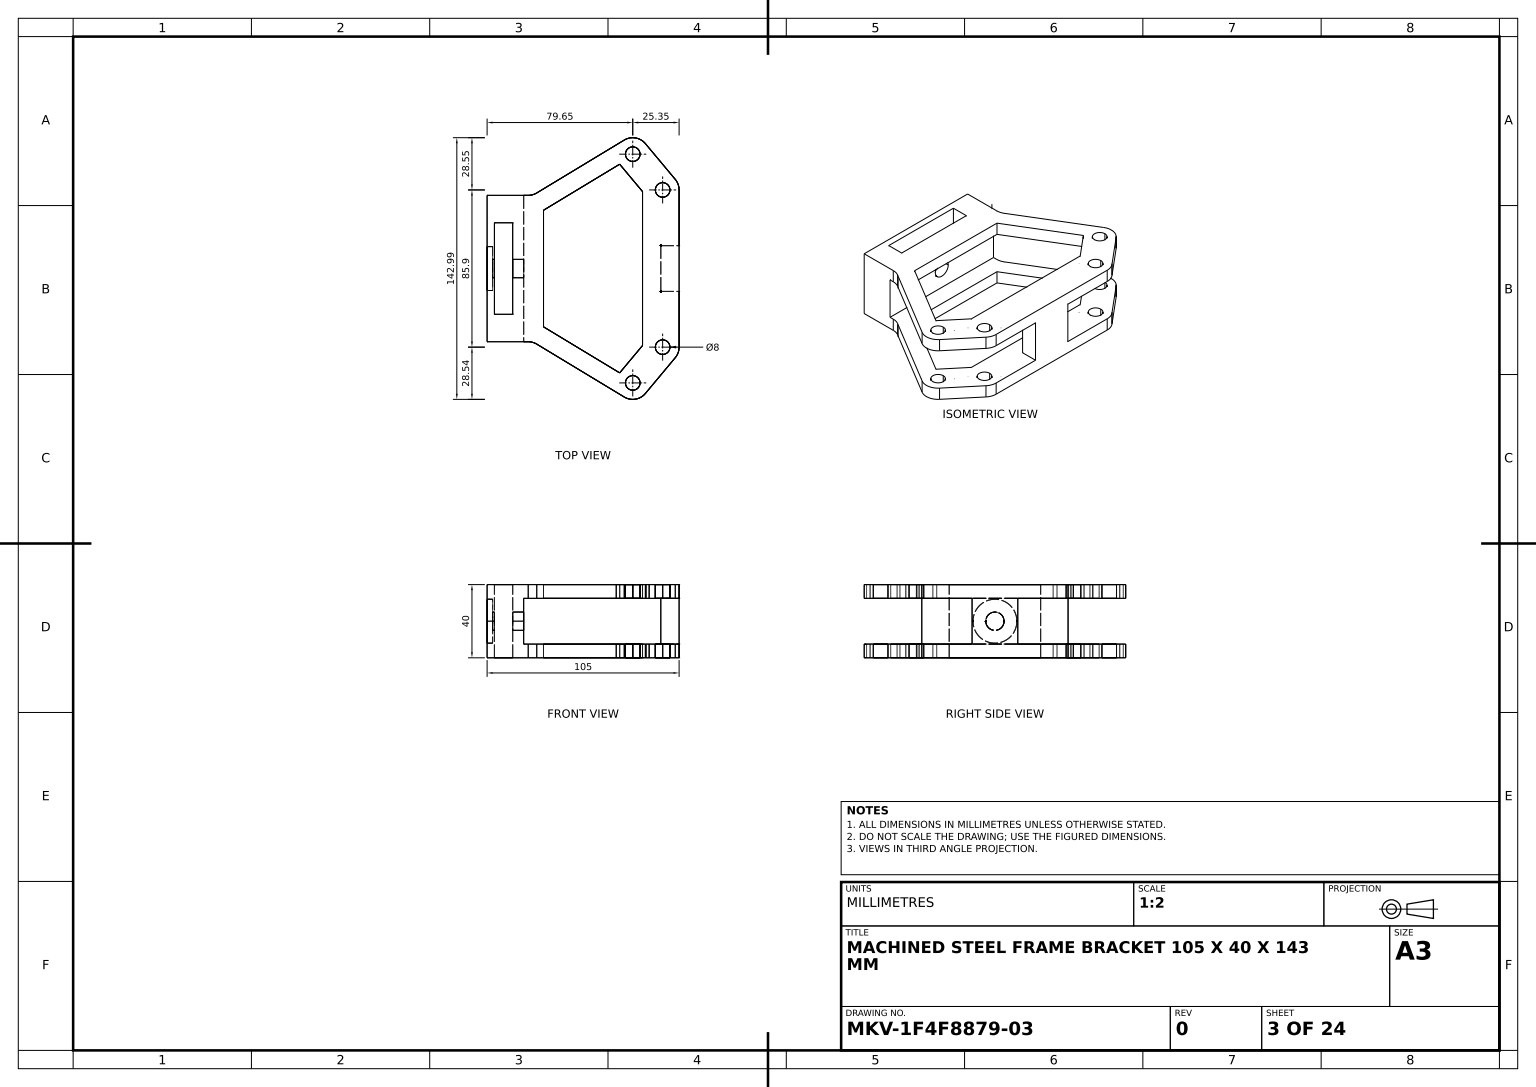
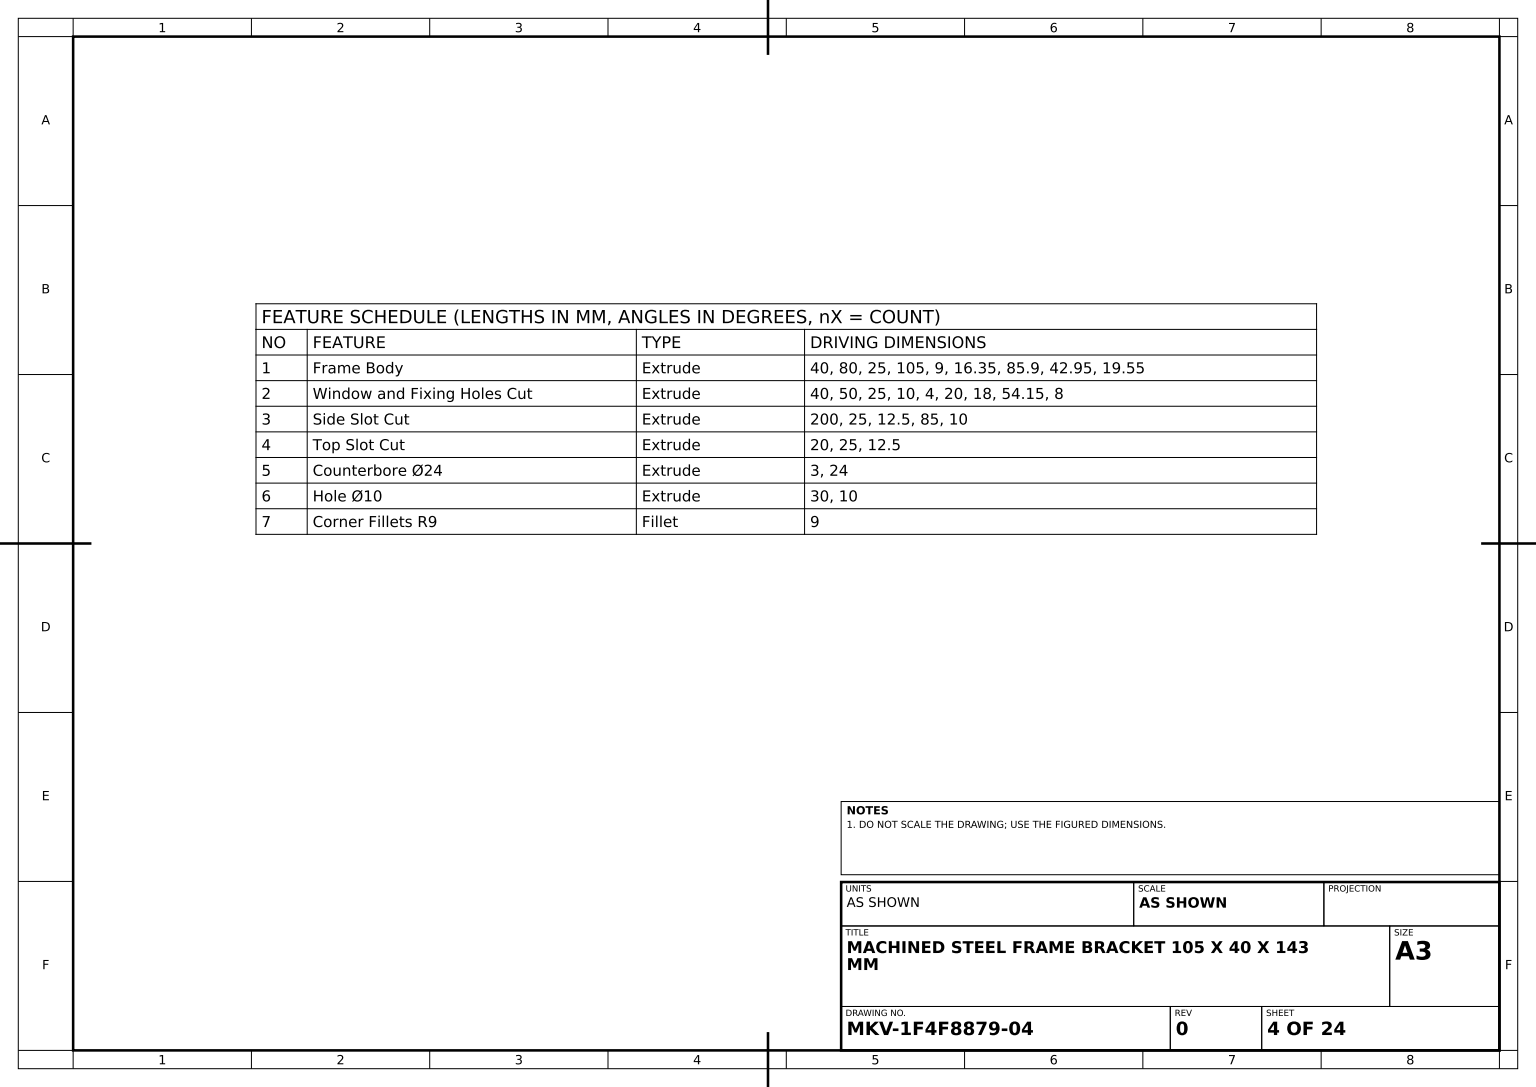
solid
v1 (27.146251,-12.5,-41.296579)
v2 (22.492509,-12.5,-40)
e1 v1 v2 CIRCLE(AX(P(22.492509,-12.5,-49),D(0,-1,0),D(0,0,-1)),9)
v3 (27.146251,-20,-41.296579)
e2 v3 v1 LINE
v4 (22.492509,-20,-40)
e3 v4 v3 CIRCLE(AX(P(22.492509,-20,-49),D(0,1,0),D(0,0,-1)),9)
e4 v2 v4 LINE
face CYL(AX(P(22.492509,20,-49),D(0,1,0),D(0,0,1)),9) rev [-e1 -e2 -e3 -e4]
v5 (95,-12.5,-12.5)
v6 (95,-12.5,12.5)
e5 v5 v6 LINE
v7 (95,12.5,12.5)
e6 v6 v7 LINE
v8 (95,12.5,-12.5)
e7 v8 v7 LINE
e8 v8 v5 LINE
face PLANE(AX(P(95,12.5,-100),D(1,0,0),D(0,1,0))) rev [e5 e6 -e7 e8]
v9 (79.65,-12.5,58.5)
v10 (79.65,-12.5,66.5)
e9 v9 v10 CIRCLE(AX(P(79.65,-12.5,62.5),D(0,1,0),D(0,0,-1)),4)
v11 (79.65,-20,66.5)
e10 v11 v10 LINE
v12 (79.65,-20,58.5)
e11 v12 v11 CIRCLE(AX(P(79.65,-20,62.5),D(0,1,0),D(0,0,1)),4)
e12 v12 v9 LINE
face CYL(AX(P(79.65,-20,62.5),D(0,1,0),D(0,0,1)),4) rev [e9 -e10 -e11 e12]
v13 (86.55385,-12.5,-68.273808)
v14 (86.55385,-20,-68.273808)
e13 v13 v14 LINE
v15 (79.65,-20,-71.5)
e14 v14 v15 CIRCLE(AX(P(79.65,-20,-62.5),D(0,1,0),D(0,0,1)),9)
v16 (79.65,-12.5,-71.5)
e15 v16 v15 LINE
e16 v16 v13 CIRCLE(AX(P(79.65,-12.5,-62.5),D(0,-1,0),D(0,0,-1)),9)
face CYL(AX(P(79.65,20,-62.5),D(0,-1,0),D(0,0,-1)),9) [e13 e14 -e15 e16]
v17 (0,0,-12)
v18 (0,0,12)
e17 v17 v18 CIRCLE(AX(P(0,0,0),D(-1,0,0),D(0,0,1)),12)
v19 (3,0,12)
e18 v19 v18 LINE
v20 (3,0,-12)
e19 v20 v19 CIRCLE(AX(P(3,0,0),D(-1,0,0),D(0,0,1)),12)
e20 v20 v17 LINE
face CYL(AX(P(3,0,0),D(-1,0,0),D(0,0,1)),12) rev [e17 -e18 -e19 e20]
v21 (86.55385,-12.5,68.273808)
v22 (74.996259,-12.5,70.203421)
e21 v21 v22 CIRCLE(AX(P(79.65,-12.5,62.5),D(0,-1,0),D(0,0,-1)),9)
v23 (74.996259,-20,70.203421)
e22 v22 v23 LINE
v24 (86.55385,-20,68.273808)
e23 v23 v24 CIRCLE(AX(P(79.65,-20,62.5),D(0,1,0),D(0,0,-1)),9)
e24 v21 v24 LINE
face CYL(AX(P(79.65,20,62.5),D(0,-1,0),D(0,0,-1)),9) [e21 e22 e23 -e24]
v25 (96,20,-46.95)
v26 (96,20,-38.95)
e25 v25 v26 CIRCLE(AX(P(96,20,-42.95),D(0,1,0),D(0,0,1)),4)
v27 (96,12.5,-38.95)
e26 v27 v26 LINE
v28 (96,12.5,-46.95)
e27 v27 v28 CIRCLE(AX(P(96,12.5,-42.95),D(0,-1,0),D(0,0,1)),4)
e28 v28 v25 LINE
face CYL(AX(P(96,-20,-42.95),D(0,1,0),D(0,0,1)),4) rev [e25 -e26 e27 e28]
v29 (105,-12.5,12.5)
e29 v6 v29 LINE
v30 (105,12.5,12.5)
e30 v29 v30 LINE
e31 v7 v30 LINE
face PLANE(AX(P(85,12.5,12.5),D(0,0,-1),D(-1,0,0))) rev [e29 e30 -e31 -e6]
e32 v11 v12 CIRCLE(AX(P(79.65,-20,62.5),D(0,1,0),D(0,0,1)),4)
e33 v10 v9 CIRCLE(AX(P(79.65,-12.5,62.5),D(0,1,0),D(0,0,-1)),4)
face CYL(AX(P(79.65,-20,62.5),D(0,1,0),D(0,0,1)),4) rev [-e12 -e32 e10 e33]
v31 (105,20,-42.95)
v32 (102.90385,20,-48.723808)
e34 v31 v32 CIRCLE(AX(P(96,20,-42.95),D(0,1,0),D(0,0,-1)),9)
v33 (105,12.5,-42.95)
e35 v31 v33 LINE
v34 (102.90385,12.5,-48.723808)
e36 v33 v34 CIRCLE(AX(P(96,12.5,-42.95),D(0,1,0),D(0,0,1)),9)
e37 v32 v34 LINE
face CYL(AX(P(96,20,-42.95),D(0,-1,0),D(0,0,-1)),9) [-e34 e35 e36 -e37]
v35 (74.996259,20,70.203421)
v36 (86.55385,20,68.273808)
e38 v35 v36 CIRCLE(AX(P(79.65,20,62.5),D(0,1,0),D(0,0,-1)),9)
v37 (74.996259,12.5,70.203421)
e39 v35 v37 LINE
v38 (86.55385,12.5,68.273808)
e40 v37 v38 CIRCLE(AX(P(79.65,12.5,62.5),D(0,1,0),D(0,0,1)),9)
e41 v36 v38 LINE
face CYL(AX(P(79.65,20,62.5),D(0,-1,0),D(0,0,-1)),9) [-e38 e39 e40 -e41]
v39 (0,20,-40)
v40 (0,-20,-40)
e42 v39 v40 LINE
v41 (22.492509,20,-40)
e43 v41 v39 LINE
v42 (22.492509,12.5,-40)
e44 v41 v42 LINE
v43 (20,12.5,-40)
e45 v42 v43 LINE
v44 (20,-12.5,-40)
e46 v43 v44 LINE
e47 v44 v2 LINE
e48 v4 v40 LINE
face PLANE(AX(P(0,20,-40),D(0,0,1),D(1,0,0))) rev [-e42 -e43 e44 e45 e46 e47 e4 e48]
v45 (79.65,20,66.5)
v46 (79.65,20,58.5)
e49 v45 v46 CIRCLE(AX(P(79.65,20,62.5),D(0,1,0),D(0,0,1)),4)
v47 (79.65,12.5,58.5)
e50 v47 v46 LINE
v48 (79.65,12.5,66.5)
e51 v47 v48 CIRCLE(AX(P(79.65,12.5,62.5),D(0,-1,0),D(0,0,1)),4)
e52 v48 v45 LINE
face CYL(AX(P(79.65,-20,62.5),D(0,1,0),D(0,0,1)),4) rev [e49 -e50 e51 e52]
v49 (79.65,20,-71.5)
v50 (79.65,12.5,-71.5)
e53 v49 v50 LINE
v51 (74.996259,12.5,-70.203421)
e54 v50 v51 CIRCLE(AX(P(79.65,12.5,-62.5),D(0,1,0),D(0,0,1)),9)
v52 (74.996259,20,-70.203421)
e55 v52 v51 LINE
e56 v49 v52 CIRCLE(AX(P(79.65,20,-62.5),D(0,1,0),D(0,0,1)),9)
face CYL(AX(P(79.65,20,-62.5),D(0,-1,0),D(0,0,-1)),9) [e53 e54 -e55 -e56]
v53 (102.90385,-20,48.723808)
e57 v24 v53 LINE
v54 (102.90385,-12.5,48.723808)
e58 v54 v53 LINE
e59 v54 v21 LINE
face PLANE(AX(P(102.90385,20,48.723808),D(-0.767094424,0,-0.641534211),D(-0.641534211,0,0.767094424))) rev [e57 -e58 e59 e24]
v55 (14,20,-25)
v56 (4,20,-25)
e60 v55 v56 LINE
v57 (4,-20,-25)
e61 v57 v56 LINE
v58 (14,-20,-25)
e62 v58 v57 LINE
e63 v58 v55 LINE
face PLANE(AX(P(4,-20,-25),D(0,0,-1),D(-1,0,0))) rev [e60 -e61 -e62 e63]
v59 (105,12.5,-12.5)
v60 (105,-12.5,-12.5)
e64 v59 v60 LINE
e65 v33 v59 LINE
v61 (105,20,42.95)
e66 v61 v31 LINE
v62 (105,12.5,42.95)
e67 v61 v62 LINE
e68 v30 v62 LINE
v63 (105,-12.5,42.95)
e69 v63 v29 LINE
v64 (105,-20,42.95)
e70 v63 v64 LINE
v65 (105,-20,-42.95)
e71 v64 v65 LINE
v66 (105,-12.5,-42.95)
e72 v66 v65 LINE
e73 v60 v66 LINE
face PLANE(AX(P(105,20,-42.95),D(-1,0,0),D(0,0,1))) rev [-e64 -e65 -e35 -e66 e67 -e68 -e30 -e69 e70 e71 -e72 -e73]
v67 (86.55385,20,-68.273808)
e74 v67 v49 CIRCLE(AX(P(79.65,20,-62.5),D(0,1,0),D(0,0,1)),9)
v68 (86.55385,12.5,-68.273808)
e75 v67 v68 LINE
e76 v68 v50 CIRCLE(AX(P(79.65,12.5,-62.5),D(0,1,0),D(0,0,1)),9)
face CYL(AX(P(79.65,20,-62.5),D(0,-1,0),D(0,0,-1)),9) [-e74 e75 e76 -e53]
v69 (30.85,-20,31.850943)
v70 (30.85,-12.5,31.850943)
e77 v69 v70 LINE
v71 (30.85,-20,-31.850943)
e78 v71 v69 LINE
v72 (30.85,-12.5,-31.850943)
e79 v71 v72 LINE
e80 v72 v70 LINE
face PLANE(AX(P(30.85,-20,-31.850943),D(-1,0,0),D(0,0,1))) rev [-e77 -e78 e79 e80]
v73 (4,0,5)
v74 (4,0,-5)
e81 v73 v74 CIRCLE(AX(P(4,0,0),D(-1,0,0),D(0,0,1)),5)
v75 (3,0,5)
e82 v73 v75 LINE
v76 (3,0,-5)
e83 v75 v76 CIRCLE(AX(P(3,0,0),D(-1,0,0),D(0,0,1)),5)
e84 v74 v76 LINE
face CYL(AX(P(33,0,0),D(-1,0,0),D(0,0,1)),5) rev [-e81 e82 e83 -e84]
v77 (85,-20,42.074035)
v78 (85,-20,-42.074035)
e85 v77 v78 LINE
v79 (85,-12.5,42.074035)
e86 v77 v79 LINE
v80 (85,-12.5,-42.074035)
e87 v79 v80 LINE
e88 v78 v80 LINE
face PLANE(AX(P(85,-20,42.074035),D(1,0,0),D(0,0,-1))) rev [-e85 e86 e87 -e88]
v81 (96,-20,-46.95)
v82 (96,-20,-38.95)
e89 v81 v82 CIRCLE(AX(P(96,-20,-42.95),D(0,1,0),D(0,0,1)),4)
e90 v82 v81 CIRCLE(AX(P(96,-20,-42.95),D(0,1,0),D(0,0,1)),4)
v83 (79.65,-20,-58.5)
v84 (79.65,-20,-66.5)
e91 v83 v84 CIRCLE(AX(P(79.65,-20,-62.5),D(0,1,0),D(0,0,1)),4)
e92 v84 v83 CIRCLE(AX(P(79.65,-20,-62.5),D(0,1,0),D(0,0,1)),4)
v85 (72.50458,-20,-57.015042)
e93 v78 v85 LINE
e94 v85 v71 LINE
v86 (72.50458,-20,57.015042)
e95 v69 v86 LINE
e96 v86 v77 LINE
v87 (4,-20,25)
e97 v57 v87 LINE
v88 (14,-20,25)
e98 v87 v88 LINE
e99 v88 v58 LINE
v89 (96,-20,46.95)
v90 (96,-20,38.95)
e100 v89 v90 CIRCLE(AX(P(96,-20,42.95),D(0,1,0),D(0,0,1)),4)
e101 v90 v89 CIRCLE(AX(P(96,-20,42.95),D(0,1,0),D(0,0,1)),4)
e102 v53 v64 CIRCLE(AX(P(96,-20,42.95),D(0,1,0),D(0,0,-1)),9)
v91 (27.146251,-20,41.296579)
e103 v91 v23 LINE
v92 (22.492509,-20,40)
e104 v91 v92 CIRCLE(AX(P(22.492509,-20,49),D(0,1,0),D(0,0,-1)),9)
v93 (0,-20,40)
e105 v93 v92 LINE
e106 v40 v93 LINE
v94 (74.996259,-20,-70.203421)
e107 v94 v3 LINE
e108 v15 v94 CIRCLE(AX(P(79.65,-20,-62.5),D(0,1,0),D(0,0,1)),9)
v95 (102.90385,-20,-48.723808)
e109 v95 v14 LINE
e110 v65 v95 CIRCLE(AX(P(96,-20,-42.95),D(0,1,0),D(0,0,-1)),9)
face PLANE(AX(P(79.65,-20,62.5),D(0,-1,0),D(0,0,-1))) [e89 e90] [e91 e92] [e11 e32] [e93 e94 e78 e95 e96 e85] [e62 e97 e98 e99] [e100 e101] [-e102 -e57 -e23 -e103 e104 -e105 -e106 -e48 e3 -e107 -e108 -e14 -e109 -e110 -e71]
e111 v74 v73 CIRCLE(AX(P(4,0,0),D(-1,0,0),D(0,0,1)),5)
v96 (4,20,25)
e112 v56 v96 LINE
e113 v87 v96 LINE
face PLANE(AX(P(4,-20,-25),D(-1,0,0),D(0,0,1))) rev [e81 e111] [-e97 e61 e112 -e113]
v97 (74.996259,-12.5,-70.203421)
e114 v97 v94 LINE
e115 v1 v97 LINE
face PLANE(AX(P(25,20,-40),D(0.517082376,0,0.855935638),D(0.855935638,0,-0.517082376))) rev [e114 e107 e2 e115]
v98 (79.65,12.5,-66.5)
v99 (79.65,20,-66.5)
e116 v98 v99 LINE
v100 (79.65,20,-58.5)
e117 v99 v100 CIRCLE(AX(P(79.65,20,-62.5),D(0,1,0),D(0,0,1)),4)
v101 (79.65,12.5,-58.5)
e118 v101 v100 LINE
e119 v101 v98 CIRCLE(AX(P(79.65,12.5,-62.5),D(0,-1,0),D(0,0,1)),4)
face CYL(AX(P(79.65,-20,-62.5),D(0,1,0),D(0,0,1)),4) rev [e116 e117 -e118 e119]
v102 (22.492509,-12.5,40)
e120 v92 v102 LINE
v103 (27.146251,-12.5,41.296579)
e121 v103 v91 LINE
e122 v102 v103 CIRCLE(AX(P(22.492509,-12.5,49),D(0,-1,0),D(0,0,-1)),9)
face CYL(AX(P(22.492509,20,49),D(0,1,0),D(0,0,1)),9) rev [-e120 -e104 -e121 -e122]
v104 (14,0,5)
v105 (14,0,-5)
e123 v104 v105 CIRCLE(AX(P(14,0,0),D(1,0,0),D(0,0,-1)),5)
v106 (20,0,5)
e124 v106 v104 LINE
v107 (20,0,-5)
e125 v107 v106 CIRCLE(AX(P(20,0,0),D(-1,0,0),D(0,-1,0)),5)
e126 v107 v105 LINE
face CYL(AX(P(33,0,0),D(-1,0,0),D(0,0,1)),5) rev [-e123 -e124 -e125 e126]
e127 v105 v104 CIRCLE(AX(P(14,0,0),D(1,0,0),D(0,0,-1)),5)
v108 (14,20,25)
e128 v88 v108 LINE
e129 v108 v55 LINE
face PLANE(AX(P(14,-20,-25),D(1,0,0),D(0,0,-1))) rev [e123 e127] [-e99 e128 e129 -e63]
v109 (30.85,20,31.850943)
v110 (72.50458,20,57.015042)
e130 v109 v110 LINE
v111 (72.50458,12.5,57.015042)
e131 v111 v110 LINE
v112 (30.85,12.5,31.850943)
e132 v111 v112 LINE
e133 v112 v109 LINE
face PLANE(AX(P(30.85,-20,31.850943),D(-0.517082376,0,0.855935638),D(0.855935638,0,0.517082376))) rev [e130 -e131 e132 e133]
e134 v76 v75 CIRCLE(AX(P(3,0,0),D(-1,0,0),D(0,0,1)),5)
face CYL(AX(P(33,0,0),D(-1,0,0),D(0,0,1)),5) rev [-e82 -e111 e84 e134]
e135 v8 v59 LINE
e136 v5 v60 LINE
face PLANE(AX(P(85,12.5,-12.5),D(0,0,1),D(1,0,0))) rev [e135 e64 -e136 -e8]
v113 (102.90385,-12.5,-48.723808)
e137 v113 v95 LINE
e138 v13 v113 LINE
face PLANE(AX(P(86.55385,20,-68.273808),D(-0.767094424,0,0.641534211),D(0.641534211,0,0.767094424))) rev [e137 e109 -e13 e138]
v114 (79.65,-12.5,-58.5)
e139 v83 v114 LINE
v115 (79.65,-12.5,-66.5)
e140 v84 v115 LINE
e141 v115 v114 CIRCLE(AX(P(79.65,-12.5,-62.5),D(0,1,0),D(0,0,-1)),4)
face CYL(AX(P(79.65,-20,-62.5),D(0,1,0),D(0,0,1)),4) rev [-e139 -e92 e140 e141]
e142 v18 v17 CIRCLE(AX(P(0,0,0),D(-1,0,0),D(0,0,1)),12)
v116 (0,20,40)
e143 v39 v116 LINE
e144 v116 v93 LINE
face PLANE(AX(P(0,20,-40),D(1,0,0),D(0,0,-1))) rev [-e142 -e17] [-e143 e42 e106 -e144]
e145 v106 v107 CIRCLE(AX(P(20,0,0),D(-1,0,0),D(0,-1,0)),5)
face CYL(AX(P(33,0,0),D(-1,0,0),D(0,0,1)),5) rev [e124 -e127 -e126 -e145]
v117 (85,12.5,42.074035)
e146 v117 v111 LINE
v118 (85,20,42.074035)
e147 v110 v118 LINE
e148 v117 v118 LINE
face PLANE(AX(P(72.50458,-20,57.015042),D(0.767094424,0,0.641534211),D(0.641534211,0,-0.767094424))) rev [e146 e131 e147 -e148]
e149 v19 v20 CIRCLE(AX(P(3,0,0),D(-1,0,0),D(0,0,1)),12)
face PLANE(AX(P(3,0,0),D(-1,0,0),D(0,0,1))) [-e83 -e134] [e149 e19]
v119 (96,20,46.95)
v120 (96,20,38.95)
e150 v119 v120 CIRCLE(AX(P(96,20,42.95),D(0,1,0),D(0,0,1)),4)
v121 (96,12.5,38.95)
e151 v121 v120 LINE
v122 (96,12.5,46.95)
e152 v121 v122 CIRCLE(AX(P(96,12.5,42.95),D(0,-1,0),D(0,0,1)),4)
e153 v122 v119 LINE
face CYL(AX(P(96,-20,42.95),D(0,1,0),D(0,0,1)),4) rev [e150 -e151 e152 e153]
e154 v114 v115 CIRCLE(AX(P(79.65,-12.5,-62.5),D(0,1,0),D(0,0,-1)),4)
face CYL(AX(P(79.65,-20,-62.5),D(0,1,0),D(0,0,1)),4) rev [-e91 e139 e154 -e140]
v123 (72.50458,-12.5,57.015042)
e155 v86 v123 LINE
e156 v123 v79 LINE
face PLANE(AX(P(72.50458,-20,57.015042),D(0.767094424,0,0.641534211),D(0.641534211,0,-0.767094424))) rev [-e96 e155 e156 -e86]
v124 (20,12.5,40)
e157 v43 v124 LINE
v125 (20,-12.5,40)
e158 v125 v124 LINE
e159 v44 v125 LINE
face PLANE(AX(P(20,12.5,-100),D(-1,0,0),D(0,-1,0))) rev [e145 e125] [-e46 e157 -e158 -e159]
v126 (96,-12.5,-46.95)
e160 v81 v126 LINE
v127 (96,-12.5,-38.95)
e161 v126 v127 CIRCLE(AX(P(96,-12.5,-42.95),D(0,1,0),D(0,0,-1)),4)
e162 v82 v127 LINE
face CYL(AX(P(96,-20,-42.95),D(0,1,0),D(0,0,1)),4) rev [e160 e161 -e162 -e89]
v128 (96,-12.5,46.95)
e163 v89 v128 LINE
v129 (96,-12.5,38.95)
e164 v128 v129 CIRCLE(AX(P(96,-12.5,42.95),D(0,1,0),D(0,0,-1)),4)
e165 v90 v129 LINE
face CYL(AX(P(96,-20,42.95),D(0,1,0),D(0,0,1)),4) rev [e163 e164 -e165 -e100]
e166 v26 v25 CIRCLE(AX(P(96,20,-42.95),D(0,1,0),D(0,0,1)),4)
e167 v120 v119 CIRCLE(AX(P(96,20,42.95),D(0,1,0),D(0,0,1)),4)
e168 v100 v99 CIRCLE(AX(P(79.65,20,-62.5),D(0,1,0),D(0,0,1)),4)
v130 (30.85,20,-31.850943)
e169 v130 v109 LINE
v131 (72.50458,20,-57.015042)
e170 v131 v130 LINE
v132 (85,20,-42.074035)
e171 v132 v131 LINE
e172 v118 v132 LINE
e173 v46 v45 CIRCLE(AX(P(79.65,20,62.5),D(0,1,0),D(0,0,1)),4)
v133 (27.146251,20,-41.296579)
e174 v52 v133 LINE
e175 v133 v41 CIRCLE(AX(P(22.492509,20,-49),D(0,-1,0),D(0,0,-1)),9)
v134 (22.492509,20,40)
e176 v116 v134 LINE
v135 (27.146251,20,41.296579)
e177 v134 v135 CIRCLE(AX(P(22.492509,20,49),D(0,-1,0),D(0,0,-1)),9)
e178 v135 v35 LINE
v136 (102.90385,20,48.723808)
e179 v36 v136 LINE
e180 v136 v61 CIRCLE(AX(P(96,20,42.95),D(0,1,0),D(0,0,-1)),9)
e181 v32 v67 LINE
e182 v96 v108 LINE
face PLANE(AX(P(79.65,20,62.5),D(0,-1,0),D(0,0,-1))) rev [-e25 -e166] [-e150 -e167] [-e168 -e117] [-e147 -e130 -e169 -e170 -e171 -e172] [-e49 -e173] [e74 e56 e174 e175 e43 e143 e176 e177 e178 e38 e179 e180 e66 e34 e181] [-e129 -e182 -e112 -e60]
v137 (27.146251,12.5,41.296579)
e183 v135 v137 LINE
e184 v137 v37 LINE
face PLANE(AX(P(74.996259,20,70.203421),D(0.517082376,0,-0.855935638),D(-0.855935638,0,-0.517082376))) rev [-e178 e183 e184 -e39]
e185 v102 v125 LINE
v138 (22.492509,12.5,40)
e186 v124 v138 LINE
e187 v138 v134 LINE
face PLANE(AX(P(0,20,40),D(0,0,-1),D(-1,0,0))) rev [e144 e105 e120 e185 e158 e186 e187 -e176]
e188 v22 v103 LINE
face PLANE(AX(P(74.996259,20,70.203421),D(0.517082376,0,-0.855935638),D(-0.855935638,0,-0.517082376))) rev [-e22 e188 e121 e103]
v139 (27.146251,12.5,-41.296579)
e189 v42 v139 CIRCLE(AX(P(22.492509,12.5,-49),D(0,1,0),D(0,0,1)),9)
e190 v139 v133 LINE
face CYL(AX(P(22.492509,20,-49),D(0,1,0),D(0,0,1)),9) rev [-e189 -e44 -e175 -e190]
e191 v70 v123 LINE
face PLANE(AX(P(30.85,-20,31.850943),D(-0.517082376,0,0.855935638),D(0.855935638,0,0.517082376))) rev [e191 -e155 -e95 e77]
e192 v129 v128 CIRCLE(AX(P(96,-12.5,42.95),D(0,1,0),D(0,0,-1)),4)
face CYL(AX(P(96,-20,42.95),D(0,1,0),D(0,0,1)),4) rev [-e163 -e101 e165 e192]
e193 v48 v47 CIRCLE(AX(P(79.65,12.5,62.5),D(0,-1,0),D(0,0,1)),4)
face CYL(AX(P(79.65,-20,62.5),D(0,1,0),D(0,0,1)),4) rev [-e52 e193 e50 e173]
e194 v127 v126 CIRCLE(AX(P(96,-12.5,-42.95),D(0,1,0),D(0,0,-1)),4)
v140 (72.50458,-12.5,-57.015042)
e195 v140 v72 LINE
e196 v80 v140 LINE
e197 v63 v54 CIRCLE(AX(P(96,-12.5,42.95),D(0,-1,0),D(0,0,-1)),9)
e198 v113 v66 CIRCLE(AX(P(96,-12.5,-42.95),D(0,-1,0),D(0,0,-1)),9)
e199 v97 v16 CIRCLE(AX(P(79.65,-12.5,-62.5),D(0,-1,0),D(0,0,-1)),9)
face PLANE(AX(P(20,-12.5,-100),D(0,-1,0),D(0,0,-1))) rev [-e161 -e194] [-e164 -e192] [-e191 -e80 -e195 -e196 -e87 -e156] [-e154 -e141] [-e59 -e197 e69 -e29 -e5 e136 e73 -e198 -e138 -e16 -e199 -e115 e1 -e47 e159 -e185 e122 -e188 -e21] [-e33 -e9]
e200 v137 v138 CIRCLE(AX(P(22.492509,12.5,49),D(0,1,0),D(0,0,1)),9)
face CYL(AX(P(22.492509,20,49),D(0,1,0),D(0,0,1)),9) rev [-e177 -e187 -e200 -e183]
e201 v34 v68 LINE
face PLANE(AX(P(86.55385,20,-68.273808),D(-0.767094424,0,0.641534211),D(0.641534211,0,0.767094424))) rev [-e181 e37 e201 -e75]
face CYL(AX(P(96,20,-42.95),D(0,-1,0),D(0,0,-1)),9) [-e137 e198 e72 e110]
e202 v85 v140 LINE
face PLANE(AX(P(72.50458,-20,-57.015042),D(-0.517082376,0,-0.855935638),D(-0.855935638,0,0.517082376))) rev [e202 e195 -e79 -e94]
e203 v51 v139 LINE
face PLANE(AX(P(25,20,-40),D(0.517082376,0,0.855935638),D(0.855935638,0,-0.517082376))) rev [-e174 e55 e203 e190]
e204 v28 v27 CIRCLE(AX(P(96,12.5,-42.95),D(0,-1,0),D(0,0,1)),4)
face CYL(AX(P(96,-20,-42.95),D(0,1,0),D(0,0,1)),4) rev [-e28 e204 e26 e166]
e205 v122 v121 CIRCLE(AX(P(96,12.5,42.95),D(0,-1,0),D(0,0,1)),4)
face CYL(AX(P(96,-20,42.95),D(0,1,0),D(0,0,1)),4) rev [e151 e167 -e153 e205]
face PLANE(AX(P(85,-20,-42.074035),D(0.767094424,0,-0.641534211),D(-0.641534211,0,-0.767094424))) rev [-e202 -e93 e88 e196]
v141 (30.85,12.5,-31.850943)
v142 (72.50458,12.5,-57.015042)
e206 v141 v142 LINE
e207 v142 v131 LINE
e208 v141 v130 LINE
face PLANE(AX(P(72.50458,-20,-57.015042),D(-0.517082376,0,-0.855935638),D(-0.855935638,0,0.517082376))) rev [e206 e207 e170 -e208]
v143 (102.90385,12.5,48.723808)
e209 v136 v143 LINE
e210 v143 v62 CIRCLE(AX(P(96,12.5,42.95),D(0,1,0),D(0,0,1)),9)
face CYL(AX(P(96,20,42.95),D(0,-1,0),D(0,0,-1)),9) [-e180 e209 e210 -e67]
e211 v98 v101 CIRCLE(AX(P(79.65,12.5,-62.5),D(0,-1,0),D(0,0,1)),4)
face CYL(AX(P(79.65,-20,-62.5),D(0,1,0),D(0,0,1)),4) rev [e168 -e116 e211 e118]
v144 (85,12.5,-42.074035)
e212 v144 v117 LINE
e213 v144 v132 LINE
face PLANE(AX(P(85,-20,42.074035),D(1,0,0),D(0,0,-1))) rev [e212 e148 e172 -e213]
face CYL(AX(P(3,0,0),D(-1,0,0),D(0,0,1)),12) rev [-e149 e18 e142 -e20]
e214 v38 v143 LINE
face PLANE(AX(P(102.90385,20,48.723808),D(-0.767094424,0,-0.641534211),D(-0.641534211,0,0.767094424))) rev [-e209 -e179 e41 e214]
face PLANE(AX(P(4,-20,25),D(0,0,1),D(1,0,0))) rev [-e128 -e98 e113 e182]
face CYL(AX(P(79.65,20,-62.5),D(0,-1,0),D(0,0,-1)),9) [e15 e108 -e114 e199]
e215 v142 v144 LINE
e216 v112 v141 LINE
face PLANE(AX(P(20,12.5,-100),D(0,1,0),D(0,0,1))) rev [-e215 -e206 -e216 -e132 -e146 -e212] [-e205 -e152] [-e51 -e193] [-e204 -e27] [-e211 -e119] [e68 -e210 -e214 -e40 -e184 e200 -e186 -e157 -e45 e189 -e203 -e54 -e76 -e201 -e36 e65 -e135 e7 e31]
face CYL(AX(P(96,20,42.95),D(0,-1,0),D(0,0,-1)),9) [e102 -e70 e197 e58]
face CYL(AX(P(96,-20,-42.95),D(0,1,0),D(0,0,1)),4) rev [-e160 -e90 e162 e194]
face PLANE(AX(P(85,-20,-42.074035),D(0.767094424,0,-0.641534211),D(-0.641534211,0,-0.767094424))) rev [e215 e213 e171 -e207]
face PLANE(AX(P(30.85,-20,-31.850943),D(-1,0,0),D(0,0,1))) rev [e169 -e133 e216 e208]
